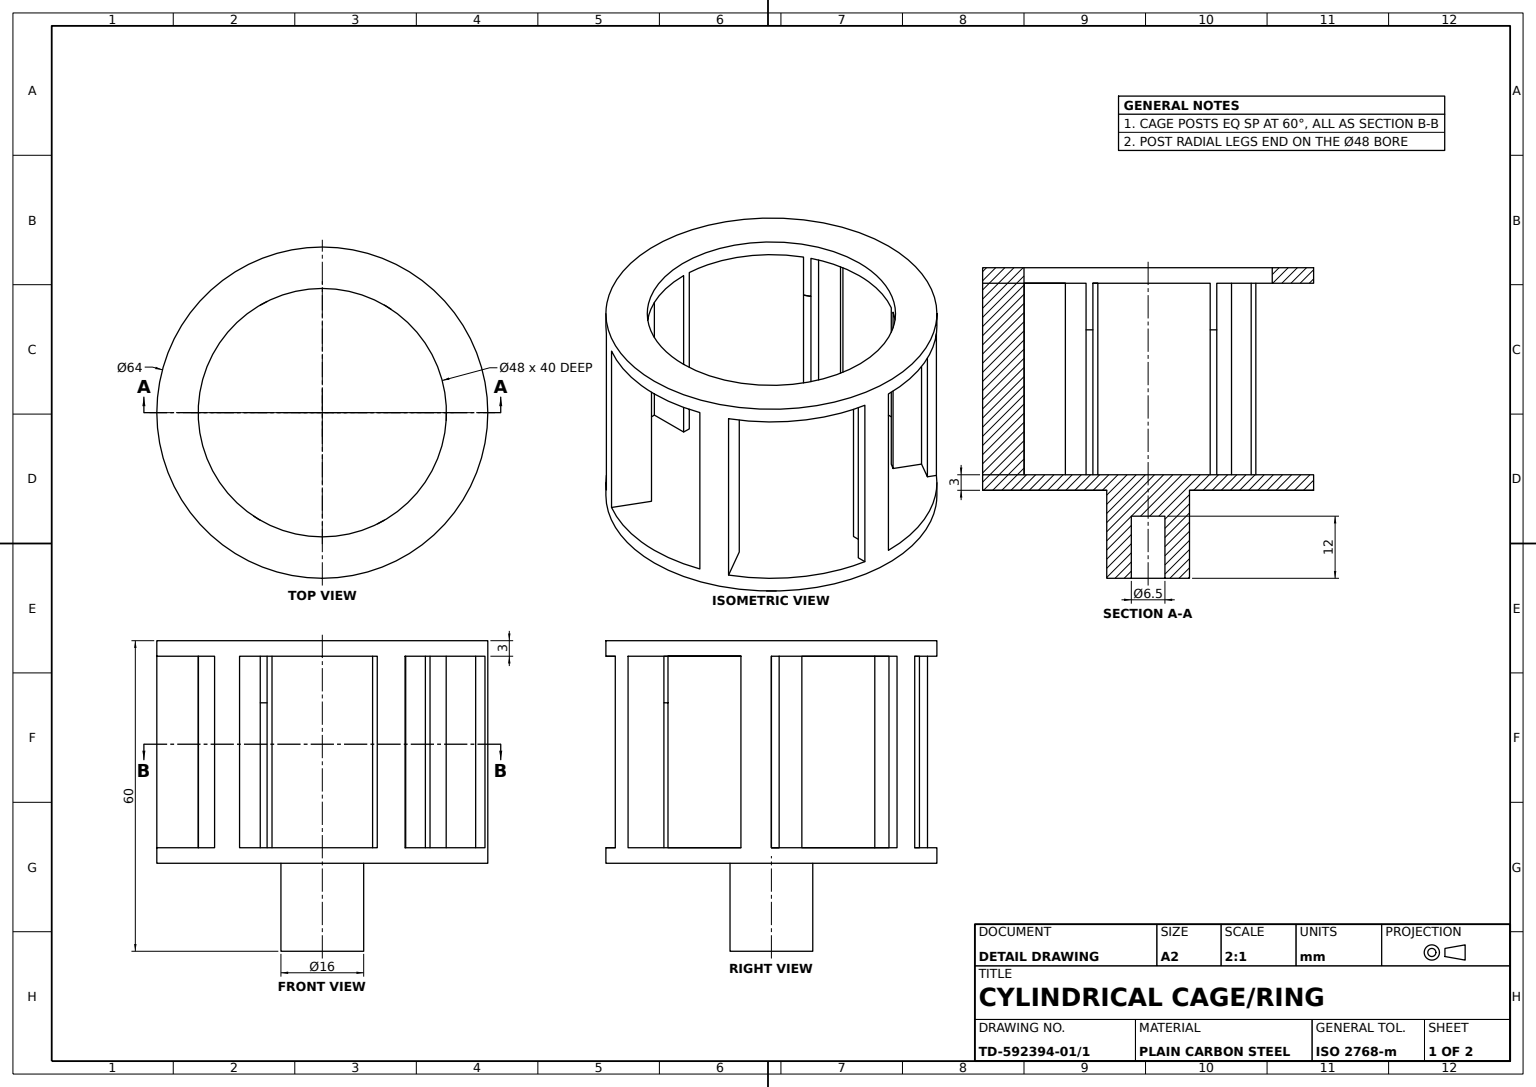
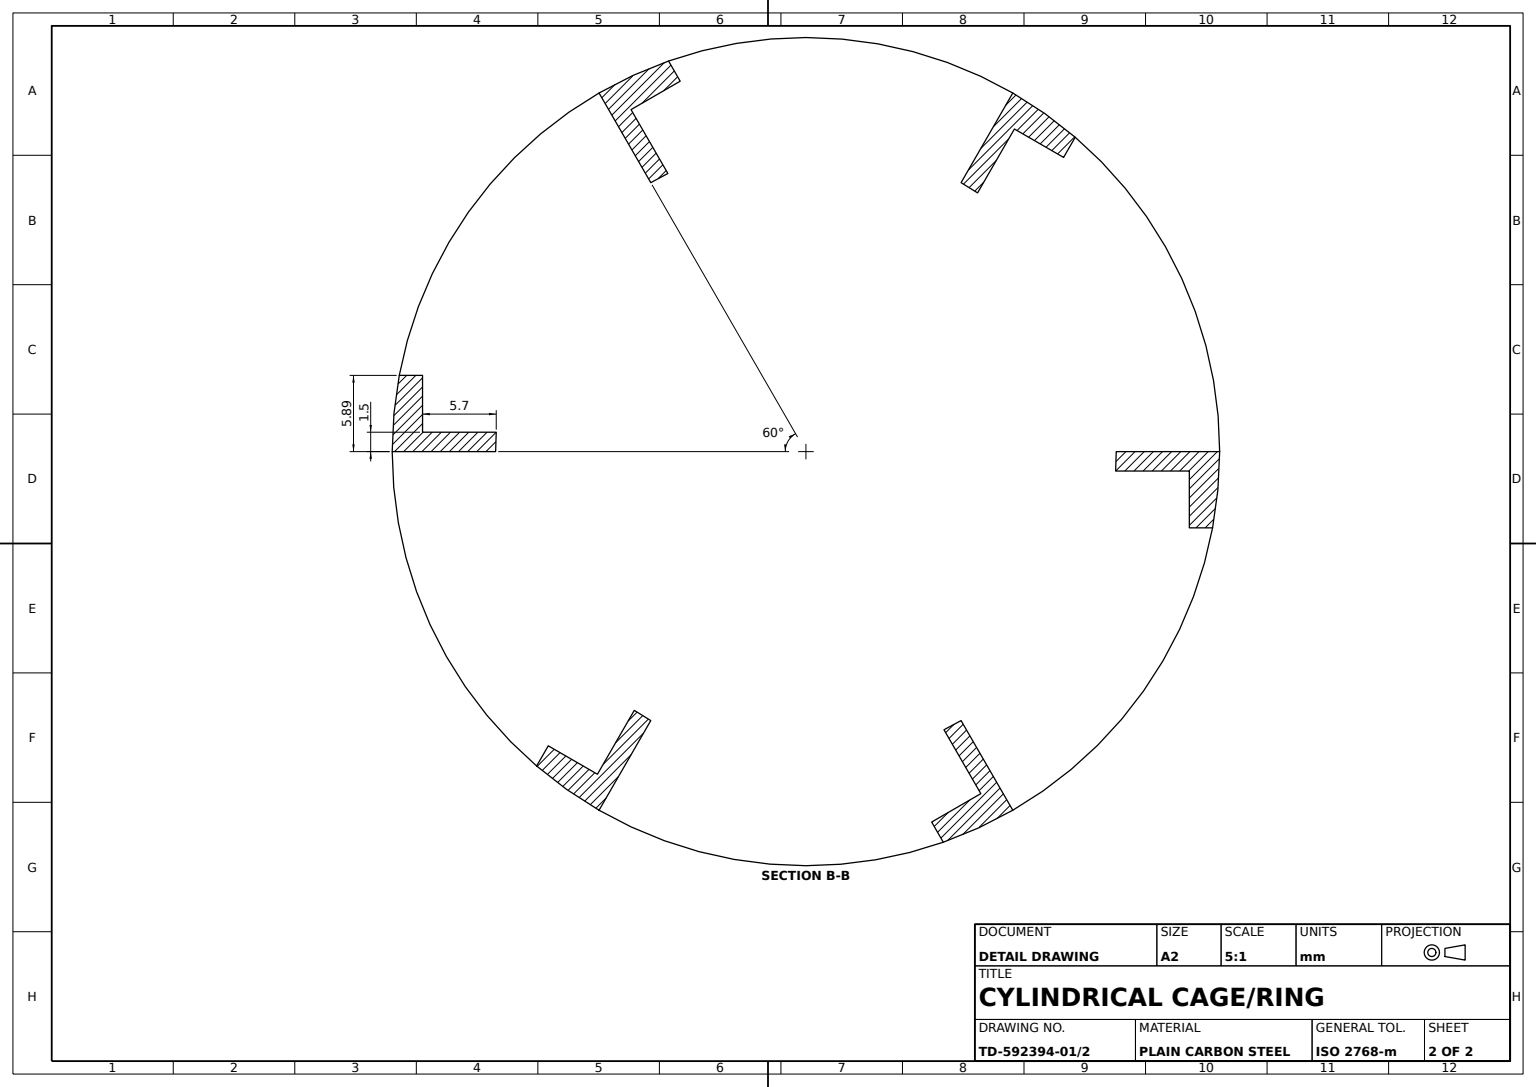
solid
v1 (23.953079,31,1.5)
v2 (23.953079,3,1.5)
e1 v1 v2 LINE
v3 (29.653079,3,1.5)
e2 v3 v2 LINE
v4 (29.653079,40,1.5)
e3 v4 v3 LINE
v5 (23.953079,40,1.5)
e4 v4 v5 LINE
e5 v5 v1 LINE
face PLANE(AX(P(0,43,1.5),D(0,0,1),D(1,0,0))) [e1 -e2 -e3 e4 e5]
v6 (10.677501,3,21.493975)
v7 (12,3,20.78461)
e6 v6 v7 LINE
v8 (16,3,27.712813)
e7 v7 v8 LINE
v9 (31.453079,3,5.890994)
e8 v8 v9 CIRCLE(AX(P(0,3,0),D(0,1,0),D(0,0,1)),32)
v10 (29.653079,3,5.890994)
e9 v9 v10 LINE
e10 v10 v3 LINE
v11 (24,3,0)
e11 v2 v11 LINE
v12 (32,3,0)
e12 v11 v12 LINE
v13 (20.82829,3,-24.293668)
e13 v12 v13 CIRCLE(AX(P(0,3,0),D(0,1,0),D(0,0,1)),32)
v14 (19.92829,3,-22.734823)
e14 v13 v14 LINE
v15 (16.125578,3,-24.93032)
e15 v14 v15 LINE
v16 (13.275578,3,-19.993975)
e16 v15 v16 LINE
v17 (12,3,-20.78461)
e17 v16 v17 LINE
v18 (16,3,-27.712813)
e18 v17 v18 LINE
v19 (0,3,-32)
e19 v18 v19 CIRCLE(AX(P(0,3,0),D(0,1,0),D(0,0,1)),32)
v20 (-10.624789,3,-30.184663)
e20 v19 v20 CIRCLE(AX(P(0,3,0),D(0,1,0),D(0,0,1)),32)
v21 (-9.724789,3,-28.625817)
e21 v20 v21 LINE
v22 (-13.527501,3,-26.43032)
e22 v21 v22 LINE
v23 (-10.677501,3,-21.493975)
e23 v22 v23 LINE
v24 (-12,3,-20.78461)
e24 v23 v24 LINE
v25 (-16,3,-27.712813)
e25 v24 v25 LINE
v26 (-31.453079,3,-5.890994)
e26 v25 v26 CIRCLE(AX(P(0,3,0),D(0,1,0),D(0,0,1)),32)
v27 (-29.653079,3,-5.890994)
e27 v26 v27 LINE
v28 (-29.653079,3,-1.5)
e28 v27 v28 LINE
v29 (-23.953079,3,-1.5)
e29 v28 v29 LINE
v30 (-24,3,0)
e30 v29 v30 CIRCLE(AX(P(0,3,0),D(0,1,0),D(0,0,1)),24)
v31 (-32,3,0)
e31 v30 v31 LINE
v32 (-20.82829,3,24.293668)
e32 v31 v32 CIRCLE(AX(P(0,3,0),D(0,1,0),D(0,0,1)),32)
v33 (-19.92829,3,22.734823)
e33 v32 v33 LINE
v34 (-16.125578,3,24.93032)
e34 v33 v34 LINE
v35 (-13.275578,3,19.993975)
e35 v34 v35 LINE
v36 (-12,3,20.78461)
e36 v35 v36 LINE
v37 (-16,3,27.712813)
e37 v36 v37 LINE
v38 (0,3,32)
e38 v37 v38 CIRCLE(AX(P(0,3,0),D(0,1,0),D(0,0,1)),32)
v39 (10.624789,3,30.184663)
e39 v38 v39 CIRCLE(AX(P(0,3,0),D(0,1,0),D(0,0,1)),32)
v40 (9.724789,3,28.625817)
e40 v39 v40 LINE
v41 (13.527501,3,26.43032)
e41 v40 v41 LINE
e42 v41 v6 LINE
face PLANE(AX(P(0,3,0),D(0,1,0),D(0,0,1))) [e6 e7 e8 e9 e10 e2 e11 e12 e13 e14 e15 e16 e17 e18 e19 e20 e21 e22 e23 e24 e25 e26 e27 e28 e29 e30 e31 e32 e33 e34 e35 e36 e37 e38 e39 e40 e41 e42]
v42 (29.653079,40,5.890994)
e43 v42 v4 LINE
v43 (31.453079,40,5.890994)
e44 v43 v42 LINE
v44 (16,40,27.712813)
e45 v44 v43 CIRCLE(AX(P(0,40,0),D(0,1,0),D(0,0,1)),32)
v45 (12,40,20.78461)
e46 v45 v44 LINE
e47 v45 v5 CIRCLE(AX(P(0,40,0),D(0,1,0),D(0,0,1)),24)
face PLANE(AX(P(0,40,0),D(0,1,0),D(0,0,1))) rev [-e43 -e44 -e45 -e46 e47 -e4]
e48 v42 v10 LINE
e49 v43 v9 LINE
face PLANE(AX(P(0,43,5.890994),D(0,0,1),D(1,0,0))) [e48 -e9 -e49 e44]
v46 (0,-5,-3.25)
v47 (0,-17,-3.25)
e50 v46 v47 LINE
v48 (0,-17,3.25)
e51 v47 v48 CIRCLE(AX(P(0,-17,0),D(0,-1,0),D(0,0,-1)),3.25)
v49 (0,-5,3.25)
e52 v49 v48 LINE
e53 v46 v49 CIRCLE(AX(P(0,-5,0),D(0,-1,0),D(0,0,-1)),3.25)
face CYL(AX(P(0,-5,0),D(0,-1,0),D(0,0,-1)),3.25) rev [e50 e51 -e52 -e53]
v50 (-10.624789,40,-30.184663)
v51 (-9.724789,40,-28.625817)
e54 v50 v51 LINE
e55 v51 v21 LINE
e56 v50 v20 LINE
face PLANE(AX(P(-10.624789,43,-30.184663),D(0.866025404,0,-0.5),D(-0.5,0,-0.866025404))) [e54 e55 -e21 -e56]
v52 (0,0,-32)
e57 v19 v52 LINE
v53 (0,0,32)
e58 v52 v53 CIRCLE(AX(P(0,0,0),D(0,1,0),D(0,0,1)),32)
e59 v38 v53 LINE
v54 (-16,40,27.712813)
e60 v54 v37 LINE
v55 (0,40,32)
e61 v54 v55 CIRCLE(AX(P(0,40,0),D(0,1,0),D(0,0,1)),32)
v56 (0,43,32)
e62 v56 v55 LINE
v57 (0,43,-32)
e63 v57 v56 CIRCLE(AX(P(0,43,0),D(0,1,0),D(0,0,1)),32)
v58 (0,40,-32)
e64 v57 v58 LINE
e65 v58 v50 CIRCLE(AX(P(0,40,0),D(0,1,0),D(0,0,1)),32)
v59 (-32,40,0)
e66 v59 v31 LINE
v60 (-20.82829,40,24.293668)
e67 v59 v60 CIRCLE(AX(P(0,40,0),D(0,1,0),D(0,0,1)),32)
e68 v60 v32 LINE
v61 (-16,40,-27.712813)
e69 v61 v25 LINE
v62 (-31.453079,40,-5.890994)
e70 v61 v62 CIRCLE(AX(P(0,40,0),D(0,1,0),D(0,0,1)),32)
e71 v62 v26 LINE
face CYL(AX(P(0,3,0),D(0,-1,0),D(0,0,-1)),32) [-e20 e57 e58 -e59 -e38 -e60 e61 -e62 -e63 e64 e65 e56] [-e66 e67 e68 -e32] [-e69 e70 e71 -e26]
v63 (-13.275578,31,19.993975)
v64 (-12,31,20.78461)
e72 v63 v64 LINE
e73 v63 v64 CIRCLE(AX(P(0,31,0),D(0,1,0),D(0,0,1)),24)
face PLANE(AX(P(0,31,0),D(0,1,0),D(0,0,1))) [-e72 e73]
v65 (12,31,-20.78461)
e74 v65 v17 LINE
v66 (12,40,-20.78461)
e75 v66 v65 LINE
v67 (16,40,-27.712813)
e76 v66 v67 LINE
e77 v67 v18 LINE
face PLANE(AX(P(0,43,0),D(-0.866025404,0,-0.5),D(-0.5,0,0.866025404))) [-e18 -e74 -e75 e76 e77]
v68 (13.275578,40,-19.993975)
v69 (13.275578,31,-19.993975)
e78 v68 v69 LINE
e79 v69 v16 LINE
v70 (16.125578,40,-24.93032)
e80 v70 v15 LINE
e81 v70 v68 LINE
face PLANE(AX(P(1.299038,43,0.75),D(0.866025404,0,0.5),D(0.5,0,-0.866025404))) [e78 e79 -e16 -e80 e81]
v71 (-29.653079,40,-1.5)
e82 v71 v28 LINE
v72 (-23.953079,40,-1.5)
e83 v71 v72 LINE
e84 v72 v29 LINE
face PLANE(AX(P(0,43,-1.5),D(0,0,-1),D(-1,0,0))) [-e82 e83 e84 -e29]
v73 (32,40,0)
e85 v73 v12 LINE
v74 (20.82829,40,-24.293668)
e86 v73 v74 CIRCLE(AX(P(0,40,0),D(0,1,0),D(0,0,1)),32)
e87 v74 v13 LINE
v75 (10.624789,40,30.184663)
e88 v55 v75 CIRCLE(AX(P(0,40,0),D(0,1,0),D(0,0,1)),32)
e89 v75 v39 LINE
e90 v53 v52 CIRCLE(AX(P(0,0,0),D(0,1,0),D(0,0,1)),32)
e91 v67 v58 CIRCLE(AX(P(0,40,0),D(0,1,0),D(0,0,1)),32)
e92 v56 v57 CIRCLE(AX(P(0,43,0),D(0,1,0),D(0,0,1)),32)
e93 v44 v8 LINE
face CYL(AX(P(0,3,0),D(0,-1,0),D(0,0,-1)),32) [-e85 e86 e87 -e13] [e62 e88 e89 -e39 e59 e90 -e57 -e19 -e77 e91 -e64 -e92] [e49 -e8 -e93 e45]
e94 v49 v46 CIRCLE(AX(P(0,-5,0),D(0,-1,0),D(0,0,-1)),3.25)
e95 v48 v47 CIRCLE(AX(P(0,-17,0),D(0,-1,0),D(0,0,-1)),3.25)
face CYL(AX(P(0,-5,0),D(0,-1,0),D(0,0,-1)),3.25) rev [-e94 e52 e95 -e50]
v76 (-10.677501,40,-21.493975)
v77 (-10.677501,31,-21.493975)
e96 v76 v77 LINE
e97 v77 v23 LINE
v78 (-13.527501,40,-26.43032)
e98 v78 v22 LINE
e99 v78 v76 LINE
face PLANE(AX(P(-13.527501,43,-26.43032),D(0.866025404,0,-0.5),D(-0.5,0,-0.866025404))) [e96 e97 -e23 -e98 e99]
v79 (13.527501,40,26.43032)
e100 v79 v41 LINE
v80 (10.677501,40,21.493975)
e101 v79 v80 LINE
v81 (10.677501,31,21.493975)
e102 v80 v81 LINE
e103 v81 v6 LINE
face PLANE(AX(P(13.527501,43,26.43032),D(-0.866025404,0,0.5),D(0.5,0,0.866025404))) [-e42 -e100 e101 e102 e103]
e104 v69 v65 CIRCLE(AX(P(0,31,0),D(0,1,0),D(0,0,1)),24)
e105 v69 v65 LINE
face PLANE(AX(P(0,31,0),D(0,1,0),D(0,0,1))) [e104 -e105]
v82 (-12,31,-20.78461)
e106 v82 v24 LINE
v83 (-12,40,-20.78461)
e107 v83 v82 LINE
e108 v83 v61 LINE
face PLANE(AX(P(-12,43,-20.78461),D(-0.866025404,0,0.5),D(0.5,0,0.866025404))) [-e106 -e107 e108 e69 -e25]
v84 (12,31,20.78461)
e109 v81 v84 LINE
e110 v81 v84 CIRCLE(AX(P(0,31,0),D(0,1,0),D(0,0,1)),24)
face PLANE(AX(P(0,31,0),D(0,1,0),D(0,0,1))) [-e109 e110]
v85 (19.92829,40,-22.734823)
e111 v85 v70 LINE
e112 v85 v14 LINE
face PLANE(AX(P(14.82654,43,-25.68032),D(-0.5,0,0.866025404),D(0.866025404,0,0.5))) [e111 e80 -e15 -e112]
v86 (-24,40,0)
e113 v86 v30 LINE
e114 v86 v59 LINE
face PLANE(AX(P(0,43,0),D(0,0,1),D(1,0,0))) [e66 -e31 -e113 e114]
v87 (-13.275578,40,19.993975)
e115 v87 v63 LINE
e116 v63 v35 LINE
v88 (-16.125578,40,24.93032)
e117 v88 v34 LINE
e118 v88 v87 LINE
face PLANE(AX(P(-1.299038,43,-0.75),D(-0.866025404,0,-0.5),D(-0.5,0,0.866025404))) [e115 e116 -e35 -e117 e118]
v89 (-29.653079,40,-5.890994)
e119 v62 v89 LINE
e120 v89 v27 LINE
face PLANE(AX(P(0,43,-5.890994),D(0,0,-1),D(-1,0,0))) [e119 e120 -e27 -e71]
v90 (9.724789,40,28.625817)
e121 v75 v90 LINE
e122 v90 v40 LINE
face PLANE(AX(P(10.624789,43,30.184663),D(-0.866025404,0,0.5),D(0.5,0,0.866025404))) [-e89 e121 e122 -e40]
e123 v77 v82 LINE
face PLANE(AX(P(-10.677501,43,-21.493975),D(0.47267903,0,0.881234665),D(0.881234665,0,-0.47267903))) [-e24 -e97 e123 e106]
e124 v64 v36 LINE
face PLANE(AX(P(-12.637789,43,20.389292),D(0.526832092,0,-0.84996938),D(-0.84996938,0,-0.526832092))) [-e116 e72 e124 -e36]
e125 v45 v84 LINE
v91 (0,40,24)
e126 v91 v80 CIRCLE(AX(P(0,40,0),D(0,1,0),D(0,0,1)),24)
v92 (0,43,24)
e127 v92 v91 LINE
v93 (0,43,-24)
e128 v92 v93 CIRCLE(AX(P(0,43,0),D(0,1,0),D(0,0,1)),24)
v94 (0,40,-24)
e129 v93 v94 LINE
e130 v66 v94 CIRCLE(AX(P(0,40,0),D(0,1,0),D(0,0,1)),24)
v95 (24,40,0)
e131 v95 v68 CIRCLE(AX(P(0,40,0),D(0,1,0),D(0,0,1)),24)
v96 (24,31,0)
e132 v95 v96 LINE
e133 v1 v96 CIRCLE(AX(P(0,31,0),D(0,1,0),D(0,0,1)),24)
face CYL(AX(P(0,43,0),D(0,-1,0),D(0,0,-1)),24) rev [-e47 e125 -e110 -e102 -e126 -e127 e128 e129 -e130 e75 -e104 -e78 -e131 e132 -e133 -e5]
face PLANE(AX(P(12.637789,43,-20.389292),D(-0.526832092,0,0.84996938),D(0.84996938,0,0.526832092))) [e74 -e17 -e79 e105]
e134 v1 v96 LINE
face PLANE(AX(P(0,31,0),D(0,1,0),D(0,0,1))) [-e134 e133]
v97 (-12,40,20.78461)
e135 v97 v64 LINE
e136 v97 v54 LINE
face PLANE(AX(P(0,43,0),D(0.866025404,0,0.5),D(0.5,0,-0.866025404))) [e60 -e37 -e124 -e135 e136]
v98 (0,-17,-8)
v99 (0,-17,8)
e137 v98 v99 CIRCLE(AX(P(0,-17,0),D(0,-1,0),D(0,0,-1)),8)
e138 v99 v98 CIRCLE(AX(P(0,-17,0),D(0,-1,0),D(0,0,-1)),8)
face PLANE(AX(P(0,-17,0),D(0,-1,0),D(0,0,-1))) [e137 e138] [-e51 -e95]
v100 (-19.92829,40,22.734823)
e139 v100 v33 LINE
e140 v100 v88 LINE
face PLANE(AX(P(-14.82654,43,25.68032),D(0.5,0,-0.866025404),D(-0.866025404,0,-0.5))) [-e34 -e139 e140 e117]
v101 (0,0,-8)
e141 v98 v101 LINE
v102 (0,0,8)
e142 v101 v102 CIRCLE(AX(P(0,0,0),D(0,-1,0),D(0,0,-1)),8)
e143 v99 v102 LINE
face CYL(AX(P(0,-17,0),D(0,1,0),D(0,0,1)),8) [-e137 e141 e142 -e143]
e144 v90 v79 LINE
e145 v97 v91 CIRCLE(AX(P(0,40,0),D(0,1,0),D(0,0,1)),24)
face PLANE(AX(P(0,40,0),D(0,1,0),D(0,0,1))) rev [-e101 -e144 -e121 -e88 -e61 -e136 e145 e126]
e146 v96 v11 LINE
e147 v95 v73 LINE
face PLANE(AX(P(0,43,0),D(0,0,-1),D(-1,0,0))) [-e12 -e146 -e132 e147 e85]
e148 v77 v82 CIRCLE(AX(P(0,31,0),D(0,1,0),D(0,0,1)),24)
face PLANE(AX(P(0,31,0),D(0,1,0),D(0,0,1))) [e148 -e123]
e149 v89 v71 LINE
face PLANE(AX(P(-29.653079,43,0),D(1,0,0),D(0,0,-1))) [-e120 e149 e82 -e28]
e150 v84 v7 LINE
face PLANE(AX(P(10.677501,43,21.493975),D(-0.47267903,0,-0.881234665),D(-0.881234665,0,0.47267903))) [e109 e150 -e6 -e103]
e151 v102 v101 CIRCLE(AX(P(0,0,0),D(0,-1,0),D(0,0,-1)),8)
face PLANE(AX(P(0,0,0),D(0,1,0),D(0,0,1))) rev [-e90 -e58] [-e151 -e142]
e152 v93 v92 CIRCLE(AX(P(0,43,0),D(0,1,0),D(0,0,1)),24)
face PLANE(AX(P(0,43,0),D(0,1,0),D(0,0,1))) [e92 e63] [-e128 -e152]
e153 v83 v72 CIRCLE(AX(P(0,40,0),D(0,1,0),D(0,0,1)),24)
face PLANE(AX(P(0,40,0),D(0,1,0),D(0,0,1))) rev [-e149 -e119 -e70 -e108 e153 -e83]
face PLANE(AX(P(12,43,20.78461),D(0.866025404,0,-0.5),D(-0.5,0,-0.866025404))) [e93 -e7 -e150 -e125 e46]
e154 v74 v85 LINE
face PLANE(AX(P(0,40,0),D(0,1,0),D(0,0,1))) rev [e131 -e81 -e111 -e154 -e86 -e147]
e155 v94 v76 CIRCLE(AX(P(0,40,0),D(0,1,0),D(0,0,1)),24)
e156 v51 v78 LINE
face PLANE(AX(P(0,40,0),D(0,1,0),D(0,0,1))) rev [e155 -e99 -e156 -e54 -e65 -e91 -e76 e130]
face PLANE(AX(P(-9.724789,43,-28.625817),D(0.5,0,0.866025404),D(0.866025404,0,-0.5))) [e98 -e22 -e55 e156]
e157 v86 v87 CIRCLE(AX(P(0,40,0),D(0,1,0),D(0,0,1)),24)
face CYL(AX(P(0,43,0),D(0,-1,0),D(0,0,-1)),24) rev [e135 -e73 -e115 -e157 e113 -e30 -e84 -e153 e107 -e148 -e96 -e155 -e129 e152 e127 -e145]
face PLANE(AX(P(29.653079,43,0),D(-1,0,0),D(0,0,1))) [-e10 -e48 e43 e3]
e158 v60 v100 LINE
face PLANE(AX(P(-5.101751,43,-2.945497),D(-0.866025404,0,-0.5),D(-0.5,0,0.866025404))) [e158 e139 -e33 -e68]
face PLANE(AX(P(0,-5,0),D(0,-1,0),D(0,0,-1))) [e53 e94]
face PLANE(AX(P(9.724789,43,28.625817),D(-0.5,0,-0.866025404),D(-0.866025404,0,0.5))) [e100 -e41 -e122 e144]
face PLANE(AX(P(0,40,0),D(0,1,0),D(0,0,1))) rev [-e114 e157 -e118 -e140 -e158 -e67]
face PLANE(AX(P(5.101751,43,2.945497),D(0.866025404,0,0.5),D(0.5,0,-0.866025404))) [-e87 e154 e112 -e14]
face PLANE(AX(P(23.97654,43,0.75),D(-0.999511121,0,-0.031265285),D(-0.031265285,0,0.999511121))) [-e11 -e1 e134 e146]
face CYL(AX(P(0,-17,0),D(0,1,0),D(0,0,1)),8) [-e141 -e138 e143 e151]
